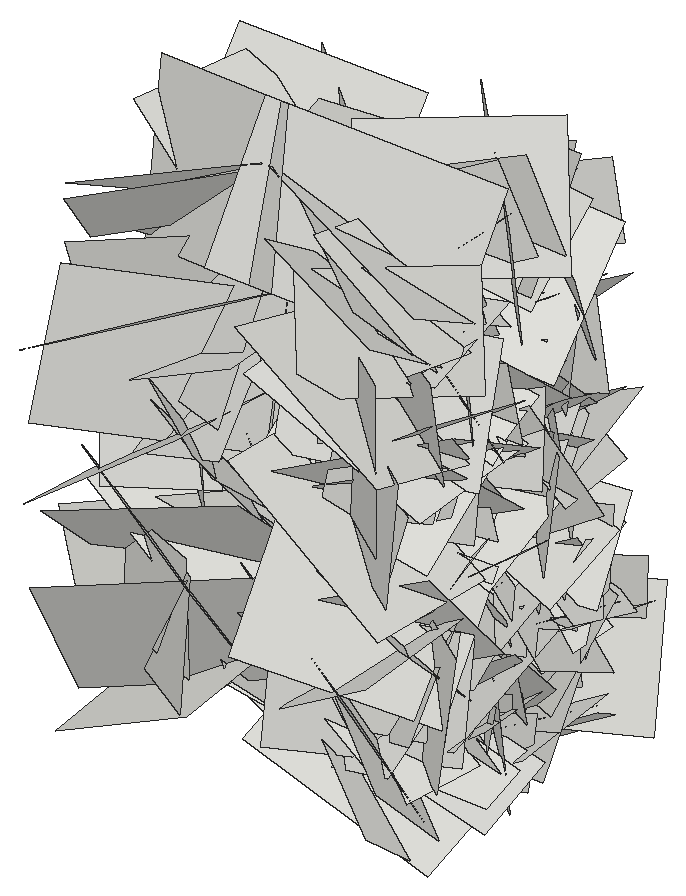
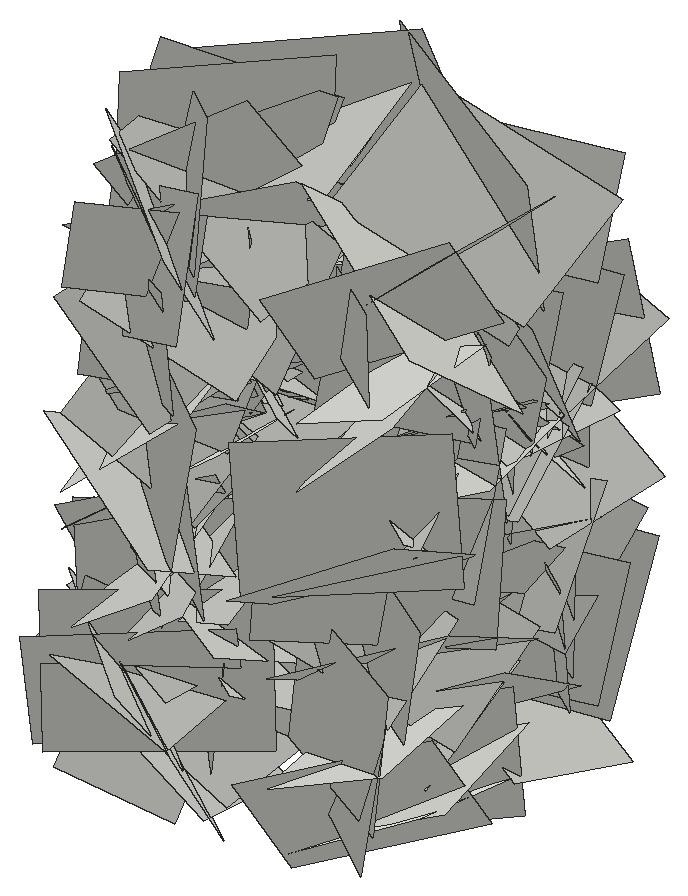
# SketchUp Ruby script. Lengths in inches.
U = 1.inch
M = Sketchup.active_model
def pt(a) = Geom::Point3d.new(a.map { |v| v * U })
def face(e, loops, mat)
  f = e.add_face(loops[0].map { |a| pt(a) })
  loops[1..].each { |l| e.add_face(l.map { |a| pt(a) }).erase! }
  f.material = f.back_material = mat if mat
  f
end
# faces: each face lists its corners as indices into pts; further lists are holes
def faces(e, pts, list, mat = nil) = list.each { |f| face(e, (f[0].is_a?(Array) ? f : [f]).map { |l| l.map { |i| pts[i] } }, mat) }
# xy, xz, yz: faces in a plane at the given z, y or x. An outline is a flat list of corners, or four numbers for a rectangle; further outlines are holes
def ring(l) = l.size == 4 ? [[l[0], l[1]], [l[2], l[1]], [l[2], l[3]], [l[0], l[3]]] : l.each_slice(2).to_a
def flat(e, list, mat, &to3) = list.each { |f| face(e, (f[0].is_a?(Array) ? f : [f]).map { |l| ring(l).map { |u, v| to3.(u, v) } }, mat) }
def xy(e, z, list, mat = nil) = flat(e, list, mat) { |x, y| [x, y, z] }
def xz(e, y, list, mat = nil) = flat(e, list, mat) { |x, z| [x, y, z] }
def yz(e, x, list, mat = nil) = flat(e, list, mat) { |y, z| [x, y, z] }
def lines(e, pts, list) = list.each { |a, b| e.add_line(pt(pts[a]), pt(pts[b])) }
# prism: a flat outline (further loops are holes) pulled along v
def prism(e, loops, v, mat = nil)
  f = face(e, loops, mat); d = Geom::Vector3d.new(v.map { |x| x * U })
  f.pushpull(f.normal.samedirection?(d) ? d.length : -d.length)
end
def box(e, o, s, mat = nil) = prism(e, [[o, [o[0] + s[0], o[1], o[2]], [o[0] + s[0], o[1] + s[1], o[2]], [o[0], o[1] + s[1], o[2]]]], [0, 0, s[2]], mat)
def at(x, y, z, deg = 0) = Geom::Transformation.translation(pt([x, y, z])) * Geom::Transformation.rotation(ORIGIN, Z_AXIS, deg.degrees)
def axes(o, x, y, z) = Geom::Transformation.new([*x, 0, *y, 0, *z, 0, *pt(o).to_a, 1])
def part(name) = M.definitions.add(name)
# library, detail: a bought-in or finely detailed component or shape, given as its bounding box
def library(name, o, s) = part(name).tap { |d| box(d.entities, o, s) }
def detail(e, o, s) = box(e.add_group.entities, o, s)
def put(e, d, t, mat = nil) = e.add_instance(d, t).tap { |i| i.material = mat if mat }
def group(e, t, mat = nil) = e.add_group.tap { |g| g.transformation = t; g.material = mat if mat }.entities
root = M.entities
c1 = part("Component\#6")
p = [[0.01,0,0],[0,3.24,4.54],[4.32,3.24,4.54],[4.33,0,0]]
faces(c1.entities,p,[[0,1,2,3]])
put(root,c1,axes([404.88,139.99,14.29],[-0.01199,-0.16574,0.68191],[0.09091,0.67656,0.16586],[-0.73829,0.086,0.00935]))
put(root,c1,axes([404.88,147.58,14.43],[0.15626,-0.88067,0.15465],[0.14549,0.17716,0.87807],[-0.93656,-0.11942,0.1622]))
put(root,c1,axes([404.88,138.3,10.21],[0.07821,-0.14386,0.79141],[0.12147,0.78851,0.13265],[-0.84394,0.10016,0.09244]))
put(root,c1,axes([400.91,142.2,15.72],[-0.2001,0.61396,-1.10583],[-0.10306,-1.12181,-0.60624],[1.33676,0.00542,-0.21228]))
put(root,c1,axes([400.91,141.25,1.55],[0.11713,-0.0063,1.0149],[-0.13715,1.01248,0.02037],[1.06704,0.13083,-0.10878]))
put(root,c1,axes([400.91,144.34,6.82],[-0.01542,0.93301,-0.17325],[0.14993,-0.1692,-0.92309],[0.99466,0.03997,0.13646]))
put(root,c1,axes([400.91,137.99,14.66],[-0.08461,-0.27233,0.9902],[0.1352,0.98287,0.28059],[1.08015,-0.14435,0.04245]))
put(root,c1,axes([400.91,142.29,19.52],[0.02505,0.60517,0.90894],[-0.1077,0.90642,-0.60085],[1.15246,0.07156,-0.07591]))
put(root,c1,axes([400.91,144.58,9.97],[0.16827,0.58944,-0.69808],[-0.0398,-0.70373,-0.60275],[0.96765,-0.13145,0.0966]))
put(root,c1,axes([404.88,139.8125,20.98],[-0.02151,0.52563,-0.34386],[0.05265,-0.34162,-0.52514],[-0.66372,-0.04413,-0.03051]))
put(root,c1,axes([404.88,142.6,14.22],[0.18899,-0.6396,-0.42028],[-0.00285,-0.43205,0.65638],[-0.81124,-0.14749,-0.10022]))
put(root,c1,axes([404.88,145.36,10.15],[0.14636,-0.64891,0.3527],[0.01811,0.36152,0.65845],[-0.78267,-0.11298,0.08119]))
put(root,c1,axes([404.88,145.42,18.19],[0.07853,-0.05807,0.70782],[0.06912,0.70921,0.05136],[-0.74963,0.05931,0.07889]))
put(root,c1,axes([400.91,146.45,10.34],[0.10559,0.05407,-0.92917],[0.0532,-0.93343,-0.04894],[0.98516,0.04461,0.10223]))
put(root,c1,axes([404.88,141.95,12.73],[0.09992,0.55515,0.3498],[-0.02862,0.35638,-0.5583],[-0.69495,0.06514,0.07329]))
put(root,c1,axes([400.91,137.63,3.85],[-0.23328,-0.07655,1.22947],[0.08564,1.24535,0.092],[1.30295,-0.09556,0.21407]))
put(root,c1,axes([404.88,139.18,13.74],[0.11062,-0.13563,-0.63299],[-0.03095,-0.6415,0.13263],[-0.6855,0.00708,-0.10814]))
put(root,c1,axes([400.91,141.92,3.18],[0.02887,1.0089,0.10446],[0.06921,0.10254,-1.00735],[1.07292,-0.03376,0.06217]))
put(root,c1,axes([400.91,138.34,13.4],[0.1901,0.66514,0.65147],[-0.02496,0.66648,-0.67398],[0.98658,-0.1113,-0.14258]))
put(root,c1,axes([400.91,138.76,9.15],[0.08107,-0.07376,-0.93469],[0.12107,-0.93007,0.08274],[0.98644,0.12021,0.06666]))
put(root,c1,axes([400.91,139.52,8.83],[0.01584,-0.12995,-1.07448],[0.00128,-1.07458,0.12998],[1.14724,0.003,0.01469]))
put(root,c1,axes([400.91,137.41,10.49],[0.17918,0.96529,0.20208],[-0.06958,0.21558,-0.97489],[1.04307,-0.15144,-0.09975]))
put(root,c1,axes([400.91,141.07,4.77],[-0.0925,1.07709,-0.24358],[0.13853,-0.23255,-1.07513],[1.16232,0.11343,0.10875]))
put(root,c1,axes([400.91,143.54,11.83],[-0.01207,0.98557,0.48784],[0.03058,0.48797,-0.98515],[1.16528,-0.0026,0.03091]))
put(root,c1,axes([404.88,142.82,6.12],[-0.04161,-0.60559,-0.03198],[0.13563,-0.03959,0.59276],[-0.62835,0.03156,0.13006]))
put(root,c1,axes([400.91,142.72,8.07],[-0.13823,0.05764,1.30603],[-0.0986,1.30878,-0.06705],[1.38223,0.09912,0.12583]))
put(root,c1,axes([400.91,138.64,15.1],[-0.05154,1.07135,-0.23626],[0.10153,-0.23144,-1.06922],[1.15847,0.06794,0.08319]))
put(root,c1,axes([400.91,138.49,4.97],[-0.13436,1.04009,0.6085],[0.04809,0.61554,-1.04268],[1.27641,0.08629,0.10334]))
put(root,c1,axes([404.88,137.29,3.46],[0.14224,0.61257,0.15159],[-0.04066,0.16261,-0.62315],[-0.66768,0.1206,0.07024]))
put(root,c1,axes([400.91,137.21,11.6875],[-0.11385,0.72886,-0.88593],[0.14818,-0.87485,-0.7367],[1.20699,0.17615,0.00688]))
put(root,c1,axes([400.91,143.17,19.13],[0.20193,0.9279,-0.28366],[0.04691,-0.29708,-0.94209],[1.02744,-0.16881,0.09877]))
put(root,c1,axes([400.91,142.88,1.98],[0.0351,0.64216,0.95117],[0.00533,0.95147,-0.64254],[1.21649,-0.02269,-0.02463]))
put(root,c1,axes([400.91,137.64,18.89],[0.26376,-0.64139,0.69016],[0.02251,0.71746,0.65911],[0.99845,0.15326,-0.19718]))
put(root,c1,axes([400.91,140.93,18.6875],[-0.10901,-0.41314,-1.06231],[0.28274,-1.04573,0.38087],[1.17466,0.21337,-0.19026]))
put(root,c1,axes([400.91,141.75,2.91],[-0.11729,-1.19784,-0.30033],[0.11289,-0.30967,1.19584],[1.30414,-0.08092,-0.13053]))
put(root,c1,axes([400.91,143.08,17.68],[-0.06532,-0.13436,-1.17102],[0.13166,-1.16683,0.12734],[1.24247,0.11658,-0.07506]))
put(root,c1,axes([400.91,140.04,10.48],[-0.03722,-1.27767,0.05021],[-0.04996,0.05148,1.27723],[1.35446,-0.03321,0.04849]))
put(root,c1,axes([400.91,140.59,7.56],[-0.03383,1.06332,0.50099],[0.10932,0.50178,-1.05842],[1.24115,-0.01522,0.10688]))
put(root,c1,axes([400.91,137.94,15.45],[-0.03401,0.89045,-0.73196],[0.17038,-0.72163,-0.88493],[1.2099,0.12665,0.10405]))
put(root,c1,axes([400.91,146.96,20.2],[-0.19126,-1.0536,-0.82739],[0.10265,-0.84293,1.05228],[1.41631,-0.08119,-0.188]))
put(root,c1,axes([400.91,139.77,22.87],[0.12093,1.26112,-0.05281],[-0.18505,-0.03675,-1.25475],[1.32509,-0.12022,-0.17041]))
put(root,c1,axes([400.91,139.44,14.86],[-0.04621,-1.16691,0.31838],[0.12643,0.31289,1.16311],[1.27589,-0.07327,-0.10372]))
put(root,c1,axes([400.91,141.48,7.17],[0.20337,0.82379,-0.77749],[-0.08888,-0.77608,-0.84298],[1.19742,-0.19752,0.06948]))
put(root,c1,axes([400.91,138.37,16.22],[0.07456,0.76169,-0.90937],[0.0504,-0.91204,-0.76025],[1.25638,-0.00862,0.08446]))
put(root,c1,axes([400.91,148.05,8.79],[0.07068,0.0827,-1.14811],[0.1221,-1.14474,-0.07576],[1.21402,0.11031,0.07447]))
put(root,c1,axes([400.91,144.3,10.94],[0.16969,-0.07735,1.18237],[-0.06112,1.19119,0.08573],[1.2545,0.0685,-0.15576]))
put(root,c1,axes([400.91,144.73,5.33],[0.04426,-1.02294,0.56209],[0.16257,0.56238,1.01208],[1.2265,-0.03763,-0.15444]))
put(root,c1,axes([400.91,141.11,14.91],[0.10517,-0.78429,-0.79452],[0.18451,-0.77703,0.78876],[1.16892,0.19321,-0.05302]))
put(root,c1,axes([400.91,134.59,13.6],[0.14779,0.17555,1.29716],[-0.16453,1.29751,-0.15892],[1.37773,0.13612,-0.15813]))
put(root,c1,axes([400.91,148.13,7.79],[0.13698,0.11741,-1.23467],[-0.05668,-1.23967,-0.12348],[1.31343,-0.06574,0.12344]))
put(root,c1,axes([400.91,139.3125,6.46],[-0.05297,-0.89114,0.82127],[0.332,0.78454,0.87035],[1.24093,-0.24794,-0.1978]))
put(root,c1,axes([400.91,142.16,14.375],[-0.02255,-1.26636,-0.09652],[0.2141,-0.09868,1.25016],[1.3291,-0.00559,-0.20302]))
put(root,c1,axes([400.91,141.32,18.93],[-0.00931,-1.12138,0.55372],[0.26786,0.54072,1.09906],[1.29833,-0.1196,-0.22278]))
put(root,c1,axes([400.91,140.96,14.21],[0.1647,-0.56811,1.02456],[0.16232,1.03452,0.5504],[1.23116,-0.0604,-0.20963]))
put(root,c1,axes([400.91,137.06,3.09],[0.11239,-0.69918,1.17187],[0.18512,1.17269,0.68387],[1.43458,-0.09655,-0.18006]))
put(root,c1,axes([400.91,141.18,23.91],[0.20239,-0.45291,-1.29893],[0.24414,-1.28235,0.48098],[1.43758,0.28153,0.10118]))
put(root,c1,axes([414.68,141.18,23.91],[-0.20239,-0.45291,-1.29893],[-0.24414,-1.28235,0.48098],[-1.43758,0.28153,0.10118]))
put(root,c1,axes([414.68,137.06,3.09],[-0.11239,-0.69918,1.17187],[-0.18512,1.17269,0.68387],[-1.43458,-0.09655,-0.18006]))
put(root,c1,axes([414.68,140.96,14.21],[-0.1647,-0.56811,1.02456],[-0.16232,1.03452,0.5504],[-1.23116,-0.0604,-0.20963]))
put(root,c1,axes([414.68,141.32,18.93],[0.00931,-1.12138,0.55372],[-0.26786,0.54072,1.09906],[-1.29833,-0.1196,-0.22278]))
put(root,c1,axes([414.68,142.16,14.375],[0.02255,-1.26636,-0.09652],[-0.2141,-0.09868,1.25016],[-1.3291,-0.00559,-0.20302]))
put(root,c1,axes([414.68,139.3125,6.46],[0.05297,-0.89114,0.82127],[-0.332,0.78454,0.87035],[-1.24093,-0.24794,-0.1978]))
put(root,c1,axes([414.68,148.13,7.79],[-0.13698,0.11741,-1.23467],[0.05668,-1.23967,-0.12348],[-1.31343,-0.06574,0.12344]))
put(root,c1,axes([414.68,134.59,13.6],[-0.14779,0.17555,1.29716],[0.16453,1.29751,-0.15892],[-1.37773,0.13612,-0.15813]))
put(root,c1,axes([414.68,141.11,14.91],[-0.10517,-0.78429,-0.79452],[-0.18451,-0.77703,0.78876],[-1.16892,0.19321,-0.05302]))
put(root,c1,axes([414.68,144.73,5.33],[-0.04426,-1.02294,0.56209],[-0.16257,0.56238,1.01208],[-1.2265,-0.03763,-0.15444]))
put(root,c1,axes([414.68,144.3,10.94],[-0.16969,-0.07735,1.18237],[0.06112,1.19119,0.08573],[-1.2545,0.0685,-0.15576]))
put(root,c1,axes([414.68,138.37,16.22],[-0.07456,0.76169,-0.90937],[-0.0504,-0.91204,-0.76025],[-1.25638,-0.00862,0.08446]))
put(root,c1,axes([414.68,141.48,7.17],[-0.20337,0.82379,-0.77749],[0.08888,-0.77608,-0.84298],[-1.19742,-0.19752,0.06948]))
put(root,c1,axes([414.68,139.44,14.86],[0.04621,-1.16691,0.31838],[-0.12643,0.31289,1.16311],[-1.27589,-0.07327,-0.10372]))
put(root,c1,axes([414.68,139.77,22.87],[-0.12093,1.26112,-0.05281],[0.18505,-0.03675,-1.25475],[-1.32509,-0.12022,-0.17041]))
put(root,c1,axes([414.68,146.96,20.2],[0.19126,-1.0536,-0.82739],[-0.10265,-0.84293,1.05228],[-1.41631,-0.08119,-0.188]))
put(root,c1,axes([414.68,137.94,15.45],[0.03401,0.89045,-0.73196],[-0.17038,-0.72163,-0.88493],[-1.2099,0.12665,0.10405]))
put(root,c1,axes([414.68,140.59,7.56],[0.03383,1.06332,0.50099],[-0.10932,0.50178,-1.05842],[-1.24115,-0.01522,0.10688]))
put(root,c1,axes([414.68,140.04,10.48],[0.03722,-1.27767,0.05021],[0.04996,0.05148,1.27723],[-1.35446,-0.03321,0.04849]))
put(root,c1,axes([414.68,143.08,17.68],[0.06532,-0.13436,-1.17102],[-0.13166,-1.16683,0.12734],[-1.24247,0.11658,-0.07506]))
put(root,c1,axes([414.68,141.75,2.91],[0.11729,-1.19784,-0.30033],[-0.11289,-0.30967,1.19584],[-1.30414,-0.08092,-0.13053]))
put(root,c1,axes([414.68,140.93,18.6875],[0.10901,-0.41314,-1.06231],[-0.28274,-1.04573,0.38087],[-1.17466,0.21337,-0.19026]))
put(root,c1,axes([414.68,137.64,18.89],[-0.26376,-0.64139,0.69016],[-0.02251,0.71746,0.65911],[-0.99845,0.15326,-0.19718]))
put(root,c1,axes([414.68,142.88,1.98],[-0.0351,0.64216,0.95117],[-0.00533,0.95147,-0.64254],[-1.21649,-0.02269,-0.02463]))
put(root,c1,axes([414.68,143.17,19.13],[-0.20193,0.9279,-0.28366],[-0.04691,-0.29708,-0.94209],[-1.02744,-0.16881,0.09877]))
put(root,c1,axes([414.68,137.21,11.6875],[0.11385,0.72886,-0.88593],[-0.14818,-0.87485,-0.7367],[-1.20699,0.17615,0.00688]))
put(root,c1,axes([410.71,137.29,3.46],[-0.14224,0.61257,0.15159],[0.04066,0.16261,-0.62315],[0.66768,0.1206,0.07024]))
put(root,c1,axes([414.68,138.49,4.97],[0.13436,1.04009,0.6085],[-0.04809,0.61554,-1.04268],[-1.27641,0.08629,0.10334]))
put(root,c1,axes([414.68,138.64,15.1],[0.05154,1.07135,-0.23626],[-0.10153,-0.23144,-1.06922],[-1.15847,0.06794,0.08319]))
put(root,c1,axes([414.68,142.72,8.07],[0.13823,0.05764,1.30603],[0.0986,1.30878,-0.06705],[-1.38223,0.09912,0.12583]))
put(root,c1,axes([410.71,142.82,6.12],[0.04161,-0.60559,-0.03198],[-0.13563,-0.03959,0.59276],[0.62835,0.03156,0.13006]))
put(root,c1,axes([414.68,143.54,11.83],[0.01207,0.98557,0.48784],[-0.03058,0.48797,-0.98515],[-1.16528,-0.0026,0.03091]))
put(root,c1,axes([414.68,141.07,4.77],[0.0925,1.07709,-0.24358],[-0.13853,-0.23255,-1.07513],[-1.16232,0.11343,0.10875]))
put(root,c1,axes([414.68,137.41,10.49],[-0.17918,0.96529,0.20208],[0.06958,0.21558,-0.97489],[-1.04307,-0.15144,-0.09975]))
put(root,c1,axes([414.68,139.52,8.83],[-0.01584,-0.12995,-1.07448],[-0.00128,-1.07458,0.12998],[-1.14724,0.003,0.01469]))
put(root,c1,axes([414.68,138.76,9.15],[-0.08107,-0.07376,-0.93469],[-0.12107,-0.93007,0.08274],[-0.98644,0.12021,0.06666]))
put(root,c1,axes([414.68,138.34,13.4],[-0.1901,0.66514,0.65147],[0.02496,0.66648,-0.67398],[-0.98658,-0.1113,-0.14258]))
put(root,c1,axes([414.68,141.92,3.18],[-0.02887,1.0089,0.10446],[-0.06921,0.10254,-1.00735],[-1.07292,-0.03376,0.06217]))
put(root,c1,axes([410.71,139.18,13.74],[-0.11062,-0.13563,-0.63299],[0.03095,-0.6415,0.13263],[0.6855,0.00708,-0.10814]))
put(root,c1,axes([414.68,137.89,18.97],[-0.02244,-0.79516,0.48934],[-0.22215,0.48102,0.77258],[-0.96443,-0.0923,-0.18934]))
put(root,c1,axes([414.68,137.63,3.85],[0.23328,-0.07655,1.22947],[-0.08564,1.24535,0.092],[-1.30295,-0.09556,0.21407]))
put(root,c1,axes([410.71,141.95,12.73],[-0.09992,0.55515,0.3498],[0.02862,0.35638,-0.5583],[0.69495,0.06514,0.07329]))
put(root,c1,axes([414.68,146.45,10.34],[-0.10559,0.05407,-0.92917],[-0.0532,-0.93343,-0.04894],[-0.98516,0.04461,0.10223]))
put(root,c1,axes([410.71,145.42,18.19],[-0.07853,-0.05807,0.70782],[-0.06912,0.70921,0.05136],[0.74963,0.05931,0.07889]))
put(root,c1,axes([410.71,145.36,10.15],[-0.14636,-0.64891,0.3527],[-0.01811,0.36152,0.65845],[0.78267,-0.11298,0.08119]))
put(root,c1,axes([410.71,142.6,14.22],[-0.18899,-0.6396,-0.42028],[0.00285,-0.43205,0.65638],[0.81124,-0.14749,-0.10022]))
put(root,c1,axes([410.71,139.8125,20.98],[0.02151,0.52563,-0.34386],[-0.05265,-0.34162,-0.52514],[0.66372,-0.04413,-0.03051]))
put(root,c1,axes([414.68,144.58,9.97],[-0.16827,0.58944,-0.69808],[0.0398,-0.70373,-0.60275],[-0.96765,-0.13145,0.0966]))
put(root,c1,axes([414.68,142.29,19.52],[-0.02505,0.60517,0.90894],[0.1077,0.90642,-0.60085],[-1.15246,0.07156,-0.07591]))
put(root,c1,axes([414.68,137.99,14.66],[0.08461,-0.27233,0.9902],[-0.1352,0.98287,0.28059],[-1.08015,-0.14435,0.04245]))
put(root,c1,axes([414.68,144.34,6.82],[0.01542,0.93301,-0.17325],[-0.14993,-0.1692,-0.92309],[-0.99466,0.03997,0.13646]))
put(root,c1,axes([414.68,141.25,1.55],[-0.11713,-0.0063,1.0149],[0.13715,1.01248,0.02037],[-1.06704,0.13083,-0.10878]))
put(root,c1,axes([414.68,142.2,15.72],[0.2001,0.61396,-1.10583],[0.10306,-1.12181,-0.60624],[-1.33676,0.00542,-0.21228]))
put(root,c1,axes([410.71,138.3,10.21],[-0.07821,-0.14386,0.79141],[-0.12147,0.78851,0.13265],[0.84394,0.10016,0.09244]))
put(root,c1,axes([410.71,147.58,14.43],[-0.15626,-0.88067,0.15465],[-0.14549,0.17716,0.87807],[0.93656,-0.11942,0.1622]))
put(root,c1,axes([410.71,139.99,14.29],[0.01199,-0.16574,0.68191],[-0.09091,0.67656,0.16586],[0.73829,0.086,0.00935]))
put(root,c1,axes([414.68,139.9,15.42],[-0.08068,-0.00169,-0.87701],[-0.08263,-0.87681,0.00845],[-0.92595,0.07839,0.07566]))
put(root,c1,axes([410.71,145.32,5.58],[0.01721,-0.24816,-0.73855],[-0.187,-0.7207,0.23828],[0.80443,-0.16223,0.07119]))
put(root,c1,axes([414.68,140.66,10.67],[0.05387,-0.70807,-1.02445],[0.25854,-0.99979,0.70312],[-1.29449,-0.22915,0.09779]))
put(root,c1,axes([414.68,141.11,17.69],[-0.01651,0.23078,-0.87547],[-0.12637,-0.8685,-0.22682],[-0.95135,0.11136,0.04532]))
put(root,c1,axes([410.71,138.56,10.4375],[-0.05239,0.37979,0.51244],[0.10197,0.51253,-0.37059],[0.66837,-0.04842,0.0967]))
put(root,c1,axes([414.68,149.05,6.52],[0.16475,-0.3536,-1.09271],[0.00842,-1.10231,0.35784],[-1.21738,-0.05548,-0.1454]))
put(root,c1,axes([414.68,142.09,4.39],[-0.13266,-0.06807,0.83796],[-0.05074,0.84639,0.06161],[-0.88972,-0.03812,-0.12846]))
put(root,c1,axes([414.68,136.25,6.15],[-0.02753,0.62765,0.83331],[0.11118,0.83092,-0.62258],[-1.10023,0.06826,-0.08377]))
put(root,c1,axes([410.71,141.82,12.65],[0.04235,0.31596,0.66399],[-0.14644,0.65635,-0.30401],[0.76557,0.10807,-0.09488]))
put(root,c1,axes([414.68,145.41,21.68],[-0.17174,-0.50133,-0.77339],[0.12403,-0.79008,0.48764],[-0.96905,-0.01227,0.19948]))
put(root,c1,axes([410.71,139.97,19.34],[-0.20036,-0.21311,0.82685],[-0.01235,0.84743,0.21575],[0.90502,-0.03562,0.186]))
put(root,c1,axes([414.68,135.11,11.54],[0.10699,0.00448,1.06975],[-0.01257,1.07444,-0.00338],[-1.13388,-0.01149,0.10098]))
put(root,c1,axes([410.71,141.75,2.2],[0.07408,-0.19814,0.56205],[0.01701,0.56632,0.19765],[0.63148,0.00798,-0.07126]))
put(root,c1,axes([414.68,137.79,2.1],[0.03475,-0.78477,0.75119],[0.11687,0.75006,0.77877],[-1.14558,0.05272,0.10224]))
put(root,c1,axes([410.71,139.2,5.38],[-0.02645,-0.5119,-0.36479],[0.13209,-0.36186,0.49927],[0.65307,0.05245,-0.11575]))
put(root,c1,axes([410.71,147.44,21.48],[0.11936,-0.32986,-0.48912],[-0.02265,-0.49991,0.33221],[0.62494,0.04489,0.10546]))
put(root,c1,axes([414.68,139.48,6.78],[-0.1397,0.74364,0.31774],[-0.04551,0.31504,-0.75514],[-0.85599,-0.13812,-0.01171]))
put(root,c1,axes([414.68,146.4375,4.35],[0.18242,-1.06895,0.55133],[0.10581,0.56772,1.06956],[-1.27052,-0.1062,0.16823]))
put(root,c1,axes([410.71,141.96,13.08],[0.07799,-0.57044,-0.33182],[-0.05167,-0.33766,0.56968],[0.69762,0.03877,0.07929]))
put(root,c1,axes([414.68,137.55,18.4],[0.05522,0.7917,0.38208],[-0.20111,0.38385,-0.76951],[-0.90986,-0.0368,0.19328]))
put(root,c1,axes([410.71,140.67,1.375],[0.09858,-0.02009,0.69473],[-0.09996,0.69407,0.03269],[0.72991,0.09776,-0.08935]))
put(root,c1,axes([410.71,143.63,3.63],[0.04495,-0.13338,0.65571],[0.00407,0.65706,0.13341],[0.70927,0.00468,-0.04233]))
put(root,c1,axes([410.71,139.35,17.19],[0.06054,-0.33637,0.61942],[-0.0607,0.61718,0.34043],[0.74468,0.07766,-0.02261]))
put(root,c1,axes([414.68,145.52,15.88],[0.20612,-0.51117,0.96001],[-0.04532,0.97089,0.52562],[-1.15198,-0.12966,0.1511]))
put(root,c1,axes([410.71,136.74,12.93],[0.11437,0.04247,0.59628],[0.02624,0.60507,-0.04758],[0.63311,-0.03275,-0.10574]))
put(root,c1,axes([410.71,142.73,15.75],[-0.26089,1.021,-0.12695],[-0.10549,-0.15355,-1.04195],[1.08548,0.23047,-0.13178]))
put(root,c1,axes([414.68,139.41,15.5],[-0.07329,-0.02436,0.98546],[0.16551,0.97513,0.03506],[-1.03171,0.15816,-0.06438]))
put(root,c1,axes([410.71,143.53,7.33],[-0.11895,-0.88372,0.009],[-0.0734,0.01784,0.88799],[0.93392,-0.11115,0.07094]))
put(root,c1,axes([414.68,142.07,24.73],[0.13514,0.30002,-0.93652],[-0.09595,-0.93677,-0.31242],[-1.03799,0.12565,-0.09305]))
put(root,c1,axes([410.71,138.58,20.36],[-0.30182,0.3301,1.08442],[-0.18064,1.09293,-0.37743],[1.1879,0.25007,0.21813]))
put(root,c1,axes([414.68,143.76,15.19],[-0.09057,0.86782,-0.29614],[0.1091,-0.28647,-0.86917],[-0.96584,-0.11373,-0.07041]))
put(root,c1,axes([414.68,139.77,3.95],[-0.11908,-0.78329,-0.0515],[-0.03618,-0.0471,0.79084],[-0.83129,0.11425,-0.02704]))
put(root,c1,axes([410.71,146.8125,4.55],[-0.17148,-0.83232,0.10491],[0.08015,0.09194,0.84603],[0.88562,-0.16948,-0.05625]))
put(root,c1,axes([414.68,145.52,18.22],[0.02537,0.1253,-0.85934],[-0.08829,-0.85537,-0.12704],[-0.91628,0.08589,-0.01155]))
put(root,c1,axes([414.68,143.66,16.18],[-0.1105,0.58717,-0.52568],[-0.01323,-0.53143,-0.59111],[-0.83529,-0.06926,0.0789]))
put(root,c1,axes([414.68,147.01,9.44],[0.18802,-1.10018,-0.17062],[0.06994,-0.16208,1.11371],[-1.17806,-0.18521,0.03889]))
put(root,c1,axes([410.71,143.33,2.25],[0.06381,-0.71847,0.0034],[-0.02834,0.00117,0.7205],[0.76106,0.06028,0.02655]))
put(root,c1,axes([414.68,144.05,16.5],[-0.02895,-0.76847,-0.41691],[0.01722,-0.41749,0.76847],[-0.92657,0.01625,0.02731]))
put(root,c1,axes([414.68,143.95,11.7],[0.02215,-0.88691,-0.38082],[0.08723,-0.37788,0.88459],[-1.0194,-0.05161,0.06742]))
put(root,c1,axes([410.71,147.56,10.64],[0.00206,-0.13591,-0.77504],[-0.03252,-0.77447,0.13573],[0.83344,-0.02988,0.00721]))
put(root,c1,axes([410.71,142.57,12.97],[-0.12959,-0.66136,0.5647],[0.03976,0.56572,0.67067],[0.92097,-0.11748,0.0505]))
put(root,c1,axes([414.68,141.85,18.04],[0.12661,-0.3078,1.12748],[0.24587,1.11705,0.28038],[-1.21422,0.1941,0.17434]))
put(root,c1,axes([410.71,147.06,19.23],[-0.16196,0.05609,-0.92604],[0.00217,-0.93849,-0.05718],[0.9834,0.01131,-0.15239]))
put(root,c1,axes([410.71,141.5625,11.54],[-0.13399,-0.80117,0.38482],[0.02481,0.38556,0.81039],[0.9418,-0.12414,0.0334]))
put(root,c1,axes([410.71,149.3125,5.88],[-0.15882,-0.57412,-0.80425],[-0.08368,-0.80389,0.58857],[1.04409,-0.15176,-0.07517]))
put(root,c1,axes([414.68,143.03,2.65],[0.18528,-0.93043,-0.12384],[-0.14778,-0.15031,0.9325],[-0.98392,-0.15263,-0.16338]))
put(root,c1,axes([410.71,141.35,5.69],[0.05421,0.52298,-0.48745],[0.04158,-0.49001,-0.52162],[0.75668,-0.01054,0.06359]))
put(root,c1,axes([414.68,145.65,3.28],[-0.1646,0.60158,-0.34623],[-0.0091,-0.35642,-0.61544],[-0.73568,-0.13018,0.08507]))
put(root,c1,axes([410.71,139.62,7.21],[-0.15609,-0.9187,-0.23757],[-0.00588,-0.23958,0.92989],[1.00583,-0.14396,-0.03143]))
put(root,c1,axes([410.71,143.17,8.1],[0.04482,0.75985,0.07181],[0.00358,0.07173,-0.76102],[0.80902,-0.04241,-0.00061]))
put(root,c1,axes([410.71,141.47,13.3125],[-0.15098,-0.93805,0.13539],[-0.00567,0.13771,0.94846],[1.00463,-0.1402,0.0257]))
put(root,c1,axes([414.68,139.94,18.75],[0.02341,-0.9115,0.17831],[0.09444,0.17962,0.90714],[-0.97996,-0.00447,0.09169]))
put(root,c1,axes([410.71,144.39,10.35],[-0.12238,0.87118,-0.30871],[-0.00416,-0.31157,-0.87778],[0.97971,0.1075,-0.04229]))
put(root,c1,axes([410.71,135.6875,17.375],[-0.11773,0.10526,0.9962],[-0.108,0.99592,-0.11659],[1.05635,0.11356,0.09911]))
put(root,c1,axes([410.71,136.7,5.12],[0.11008,0.58852,-0.4619],[-0.03608,-0.46213,-0.59646],[0.7922,-0.10282,0.03702]))
put(root,c1,axes([414.68,147.32,10.4375],[0.06119,-0.47987,-0.75245],[0.01649,-0.75336,0.48165],[-0.94584,-0.04418,-0.04028]))
